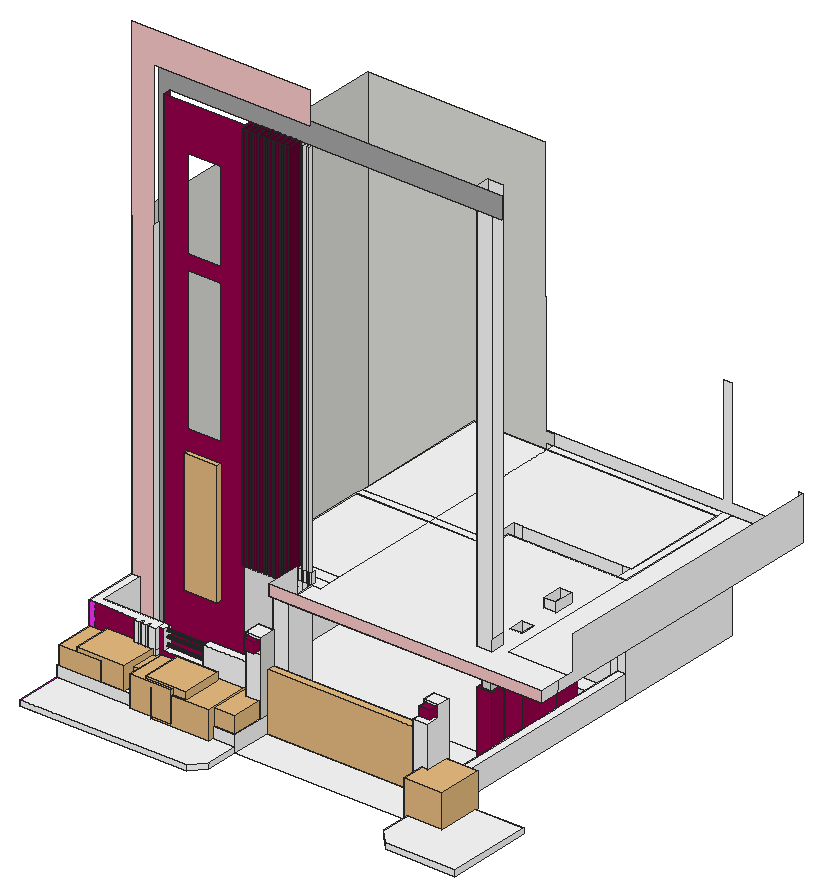
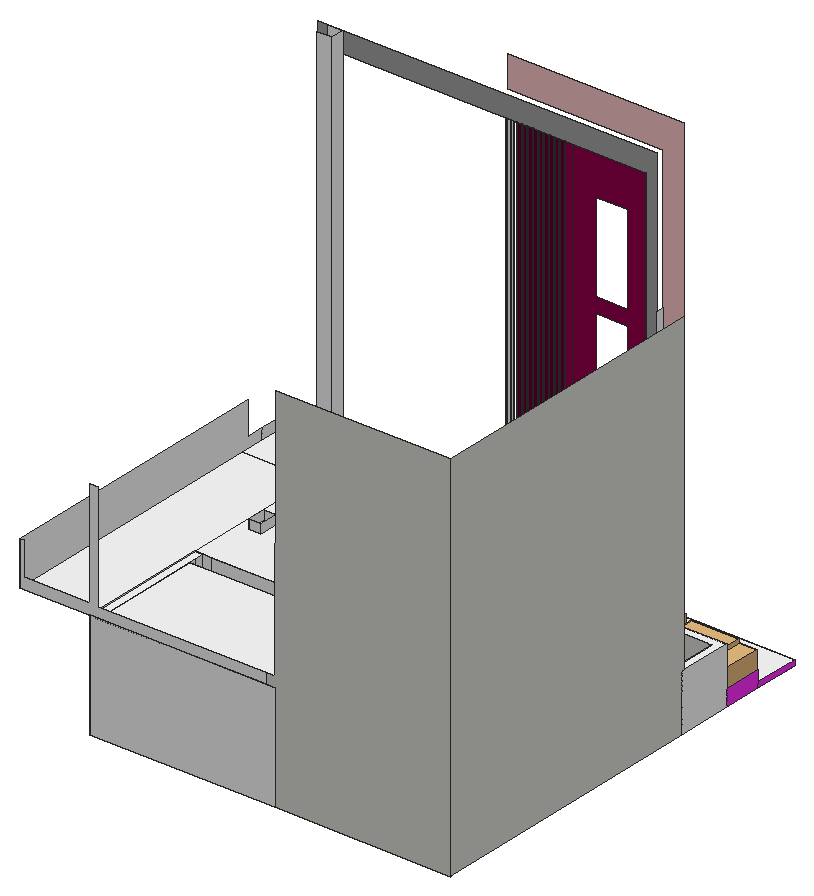
# SketchUp Ruby script. Lengths in inches.
U = 1.inch
M = Sketchup.active_model
def pt(a) = Geom::Point3d.new(a.map { |v| v * U })
def face(e, loops, mat)
  f = e.add_face(loops[0].map { |a| pt(a) })
  loops[1..].each { |l| e.add_face(l.map { |a| pt(a) }).erase! }
  f.material = f.back_material = mat if mat
  f
end
# faces: each face lists its corners as indices into pts; further lists are holes
def faces(e, pts, list, mat = nil) = list.each { |f| face(e, (f[0].is_a?(Array) ? f : [f]).map { |l| l.map { |i| pts[i] } }, mat) }
# xy, xz, yz: faces in a plane at the given z, y or x. An outline is a flat list of corners, or four numbers for a rectangle; further outlines are holes
def ring(l) = l.size == 4 ? [[l[0], l[1]], [l[2], l[1]], [l[2], l[3]], [l[0], l[3]]] : l.each_slice(2).to_a
def flat(e, list, mat, &to3) = list.each { |f| face(e, (f[0].is_a?(Array) ? f : [f]).map { |l| ring(l).map { |u, v| to3.(u, v) } }, mat) }
def xy(e, z, list, mat = nil) = flat(e, list, mat) { |x, y| [x, y, z] }
def xz(e, y, list, mat = nil) = flat(e, list, mat) { |x, z| [x, y, z] }
def yz(e, x, list, mat = nil) = flat(e, list, mat) { |y, z| [x, y, z] }
def lines(e, pts, list) = list.each { |a, b| e.add_line(pt(pts[a]), pt(pts[b])) }
# prism: a flat outline (further loops are holes) pulled along v
def prism(e, loops, v, mat = nil)
  f = face(e, loops, mat); d = Geom::Vector3d.new(v.map { |x| x * U })
  f.pushpull(f.normal.samedirection?(d) ? d.length : -d.length)
end
def box(e, o, s, mat = nil) = prism(e, [[o, [o[0] + s[0], o[1], o[2]], [o[0] + s[0], o[1] + s[1], o[2]], [o[0], o[1] + s[1], o[2]]]], [0, 0, s[2]], mat)
def at(x, y, z, deg = 0) = Geom::Transformation.translation(pt([x, y, z])) * Geom::Transformation.rotation(ORIGIN, Z_AXIS, deg.degrees)
def axes(o, x, y, z) = Geom::Transformation.new([*x, 0, *y, 0, *z, 0, *pt(o).to_a, 1])
def part(name) = M.definitions.add(name)
# library, detail: a bought-in or finely detailed component or shape, given as its bounding box
def library(name, o, s) = part(name).tap { |d| box(d.entities, o, s) }
def detail(e, o, s) = box(e.add_group.entities, o, s)
def put(e, d, t, mat = nil) = e.add_instance(d, t).tap { |i| i.material = mat if mat }
def group(e, t, mat = nil) = e.add_group.tap { |g| g.transformation = t; g.material = mat if mat }.entities
root = M.entities
M.materials.add("A01_Blush_Petal").color = [255, 204, 204]
M.materials.add("Glass_Basic_01").color = [161, 173, 186]
M.materials["Glass_Basic_01"].alpha = 0.25
M.materials.add("K04_Fuchsia_Dream").color = [255, 49, 255]
M.materials.add("L07_Raspberry_Rush").color = [153, 0, 76]
M.materials.add("L08_Velvet_Rose").color = [102, 0, 51]
M.materials.add("M00_Soft_Cloud").color = [255, 255, 255]
M.materials.add("M03_Pewter_Shine").color = [168, 168, 168]
c1 = library("Muhlenbergia dubia 005",[-26.08,-26.3,-0.58],[52.94,50.81,30.73])
c2 = library("Dalea purpurea 005",[-20.94,-21.11,-0.48],[43.54,46.19,36.21])
c3 = library("Sorghum bicolor 003",[-47.6,-43.14,-0.43],[91.82,88.31,82.26])
c4 = library("Door Unit 600mm 300 029",[-15.84,-6.47,-0.18],[31.69,12.97,85.87])
c5 = library("Gate 243 004",[-115.8,-1.69,0],[231.6,3.38,71.78])
c6 = library("Window 109 024",[-19.35,-1.51,-0.23],[38.7,3.02,80.98])
c7 = library("Scabiosa atropurpurea 007",[-28.01,-27.9375,-1.21],[55.43,54.4,41.93])
c8 = library("Group\#30",[0,0,0],[77.46,3.16,80.98])
c9 = library("Window 109 023",[-16.24,-1.39,-0.03],[32.48,2.78,89.27])
xy(root,0,[[199,95.57,377.49,104.57]])
xy(root,0,[[1,0,1,51.18,199,51.18,199,14.31,186.11,0],[1,51.18,199,51.18,199,95.57,193,95.57,193,57.18,7,57.18,7,95.57,1,95.57],[199,51.18,391.74,51.18,391.74,75.08,377.49,75.08,377.49,95.57,199,95.57],[7,57.18,193,57.18,193,86.8,182.05,86.8,182.05,95.57,78.09,95.57,78.09,91.57,69.69,91.57,69.69,95.57,67.875,95.57,67.875,91.57,61.72,91.57,61.72,95.57,59.82,95.57,59.82,91.57,53.61,91.57,53.61,95.57,7,95.57],[397.74,57.18,423.32,89.57],
  [394.03,95.57,405.98,104.57],[10,104.57,396.98,104.57,396.98,153.91,199,153.91,199,125.3,182.05,125.3,182.05,153.91,136,153.91,136,145.91,127,145.91,127,154.91,37,154.91,37,145.91,28,145.91,28,162.91,25,162.91,25,155.3,10,155.3],[182.05,125.3,199,153.91],[28,145.91,37,162.91],[[127,145.91,136,145.91,136,153.91,182.05,153.91,182.05,158.3,199,158.3,199,153.91,396.98,153.91,396.98,184.56,127,184.56],[377.49,163.42,394.03,178.61]],
  [182.05,153.91,199,158.3],[127,184.56,396.98,184.56,396.98,202.8,377.49,202.8,377.49,225.36,396.98,225.36,396.98,250.62,377.49,250.62,377.49,277.78,396.98,277.78,396.98,309.21,127,309.21],[275.24,309.21,396.98,318.21],[127,318.21,136,318.21,136,464.39,257.24,464.39,257.24,318.21,266.24,318.21,266.24,473.39,127,473.39],[136,318.21,257.24,464.39],
  [266.24,354.24,275.24,354.24,275.24,464.39,387.98,464.39,387.98,354.24,396.98,354.24,396.98,473.39,266.24,473.39],[275.24,354.24,387.98,464.39]],"M00_Soft_Cloud")
xy(root,5.18,[[22.22,93.47,50.11,95.57]],"M00_Soft_Cloud")
xy(root,5.26,[[134.27,91.57,178.26,95.57]],"L07_Raspberry_Rush")
xy(root,6,[[1,0,186.11,0,199,14.31,199,51.18,1,51.18],[407.54,0,484.64,0,484.64,95.57,429.32,95.57,429.32,51.18,391.74,51.18,391.74,17.29]],"M00_Soft_Cloud")
xy(root,6.4375,[[275.24,318.21,396.98,335.38]],"M00_Soft_Cloud")
xy(root,9.9,[[134.27,91.57,178.26,95.57]],"L07_Raspberry_Rush")
xy(root,10.95,[[22.22,93.47,50.11,95.57]],"M00_Soft_Cloud")
xy(root,18,[[1,51.18,199,51.18,199,86.8,193,86.8,193,57.18,7,57.18,7,95.57,1,95.57],[[391.74,51.18,429.32,51.18,429.32,95.57,394.03,95.57,394.03,75.08,391.74,75.08],[397.74,57.18,423.32,89.57]],[193,86.8,199,95.57]],"M00_Soft_Cloud")
xy(root,26.96,[[396.98,104.57,405.98,335.38]],"M00_Soft_Cloud")
xy(root,42.23,[[84.75,95.57,128.05,104.57]],"M00_Soft_Cloud")
xy(root,63.54,[[53.61,91.57,59.82,91.57,59.82,95.57,61.72,95.57,61.72,91.57,67.875,91.57,67.875,95.57,69.69,95.57,69.69,91.57,78.09,91.57,78.09,104.57,10,104.57,10,155.3,1,155.3,1,95.57,53.61,95.57],[78.09,95.57,84.75,104.57],[128.05,95.57,182.05,104.57]],"M00_Soft_Cloud")
xy(root,79.13,[[[377.49,163.42,394.03,178.61],[380.49,166.42,391.03,175.61]],[[377.49,202.8,396.98,225.36],[380.49,205.8,393.98,222.36]],[[377.49,250.62,396.98,277.78],[380.49,253.62,393.98,274.78]]],"L07_Raspberry_Rush")
xy(root,84.98,[[184.73,80.77,196.3125,86.8]],"L07_Raspberry_Rush")
xy(root,86.2,[[377.49,75.08,394.03,89.57]],"M00_Soft_Cloud")
xy(root,88.03,[[380.2,80.3125,392.08,89.57]],"L07_Raspberry_Rush")
xy(root,96.56,[[184.73,80.77,196.3125,86.8]],"L07_Raspberry_Rush")
xy(root,97.59,[[380.2,80.3125,392.08,89.57]],"L07_Raspberry_Rush")
xy(root,99.42,[[182.05,86.8,199,104.57],[377.49,89.57,394.03,104.57]],"M00_Soft_Cloud")
xy(root,120,[[182.05,119.76,208,125.3],[[208,119.76,484.6,119.76,484.6,171.91,405.98,171.91,405.98,335.38,275.24,335.38,275.24,309.21,208,309.21,208,158.3,199,158.3,199,125.3,208,125.3],[377.49,163.42,394.03,178.61],[380.49,205.8,393.98,222.36]],[129,148,133,148,133,162.91,135,162.91,135,148,139,148,139,162.91,141,162.91,141,148,145,148,145,162.91,147,162.91,147,148,151,148,151,162.91,153,162.91,153,148,157,148,157,162.91,159,162.91,159,148,163,148,163,162.91,165,162.91,165,148,169,148,169,162.91,171,162.91,171,148,175,148,175,162.91,177,162.91,177,148,181,148,181,162.91,198,162.91,198,158.3,208,158.3,208,171.91,127,171.91,127,162.91,129,162.91],[183,158.3,187,162.91],[189,158.3,193,162.91],
  [195,158.3,198,162.91],[[377.49,163.42,394.03,178.61],[380.49,166.42,391.03,175.61]],[127,171.91,208,184.56],[405.98,171.91,484.6,482.39],[127,184.56,208,309.21],
  [127,309.21,208,318.21],[208,309.21,266.24,318.21],[127,318.21,208,473.39],[208,318.21,266.24,318.21,266.24,354.24,396.98,354.24,396.98,473.39,208,473.39],[396.98,335.38,405.98,482.39],
  [208,473.39,396.98,482.39]],"M00_Soft_Cloud")
xz(root,0,[[1,0,186.11,6],[407.54,0,484.64,6]],"M00_Soft_Cloud")
xz(root,51.18,[[1,6,199,18],[391.74,6,429.32,18]],"M00_Soft_Cloud")
xz(root,57.18,[[7,0,193,18],[397.74,0,423.32,18]],"M00_Soft_Cloud")
xz(root,75.08,[[377.49,0,391.74,0,391.74,18,394.03,18,394.03,86.2,377.49,86.2]],"M00_Soft_Cloud")
xz(root,80.3125,[[380.2,88.03,392.08,97.59]],"L07_Raspberry_Rush")
xz(root,80.77,[[184.73,84.98,196.3125,96.56]],"L07_Raspberry_Rush")
xz(root,86.8,[[182.05,0,193,0,193,18,199,18,199,82.29,182.05,82.29],[[182.05,82.29,199,99.25],[184.73,84.98,196.3125,96.56]],[182.05,99.25,199,99.42]],"M00_Soft_Cloud")
xz(root,89.57,[[397.74,0,405.98,18],[405.98,0,423.32,18],[377.49,86.2,394.03,86.2,394.03,88.03,380.2,88.03,380.2,97.59,394.03,97.59,394.03,99.42,377.49,99.42],[392.08,88.03,394.03,97.59]],"M00_Soft_Cloud")
xz(root,91.57,[[134.27,5.26,178.26,9.9]],"L07_Raspberry_Rush")
xz(root,91.57,[[53.61,0,59.82,63.54],[61.72,0,67.875,63.54],[69.69,0,78.09,63.54]],"M00_Soft_Cloud")
xz(root,93.47,[[22.22,5.18,50.11,10.95]],"M00_Soft_Cloud")
xz(root,95.57,[[1,0,7,18],[1,18,7,63.54]],"K04_Fuchsia_Dream")
xz(root,95.57,[[[7,0,53.61,63.54],[22.22,5.18,50.11,10.95]],[78.09,0,128.05,42.23],[78.09,42.23,84.75,63.54]],"L07_Raspberry_Rush")
xz(root,95.57,[[59.82,0,61.72,63.54],[67.875,0,69.69,63.54],[[128.05,0,182.05,63.54],[134.27,5.26,178.26,9.9]],[193,0,199,18],[394.03,0,429.32,18],
  [429.32,0,484.64,6]],"M00_Soft_Cloud")
xz(root,104.57,[[10,0,10,63.54,84.75,63.54,84.75,42.23,128.05,42.23,128.05,63.54,182.05,63.54,182.05,99.42,199,99.42,199,0],[377.49,0,394.03,99.42]])
xz(root,104.57,[[394.03,0,396.98,26.96],[396.98,0,405.98,26.96]],"M00_Soft_Cloud")
xz(root,119.76,[[182.05,120,484.6,132]],"A01_Blush_Petal")
xz(root,125.3,[[182.05,0,199,120]],"M00_Soft_Cloud")
xz(root,148,[[129,120,133,554.29],[135,120,139,554.29],[141,120,145,554.29],[147,120,151,554.29],[153,120,157,554.29],
  [159,120,163,554.29],[165,120,169,554.29],[171,120,175,554.29],[177,120,181,554.29]],"L08_Velvet_Rose")
xz(root,154.91,[[[37,0,127,554.29],[63.82,229.87,100.49,387.8125],[63.82,71.93,100.49,208.3],[63.82,404,100.49,504.8]]],"L07_Raspberry_Rush")
xz(root,155.3,[[10,0,25,0,25,578.29,199,578.29,199,614.29,1,614.29,1,63.54,10,63.54]],"A01_Blush_Petal")
xz(root,158.3,[[182.05,0,183,132],[183,0,187,120],[187,0,189,132],[189,0,193,120],[193,0,195,132],
  [195,0,198,120],[198,0,199,120],[183,120,187,132],[189,120,193,132],[195,120,198,132]],"M00_Soft_Cloud")
xz(root,162.91,[[127,120,129,554.29],[133,120,135,554.29],[139,120,141,554.29],[145,120,147,554.29],[151,120,153,554.29],
  [157,120,159,554.29],[163,120,165,554.29],[169,120,171,554.29],[175,120,177,554.29],[181,120,183,554.29],
  [187,120,189,554.29],[193,120,195,554.29]],"M00_Soft_Cloud")
xz(root,162.91,[[25,0,37,0,37,554.29,405.98,554.29,405.98,578.29,25,578.29]],"M03_Pewter_Shine")
xz(root,163.42,[[377.49,0,394.03,79.13]],"L07_Raspberry_Rush")
xz(root,163.42,[[377.49,120,394.03,578.29]],"M00_Soft_Cloud")
xz(root,166.42,[[380.49,79.13,391.03,120]])
xz(root,175.61,[[380.49,79.13,391.03,120]])
xz(root,178.61,[[377.49,0,394.03,79.13]],"L07_Raspberry_Rush")
xz(root,178.61,[[377.49,120,394.03,578.29]],"M00_Soft_Cloud")
xz(root,202.8,[[377.49,0,396.98,79.13]],"L07_Raspberry_Rush")
xz(root,205.8,[[380.49,79.13,393.98,120]],"M00_Soft_Cloud")
xz(root,222.36,[[380.49,79.13,393.98,120]],"M00_Soft_Cloud")
xz(root,225.36,[[377.49,0,396.98,79.13]],"L07_Raspberry_Rush")
xz(root,250.62,[[377.49,0,396.98,79.13]],"L07_Raspberry_Rush")
xz(root,253.62,[[380.49,79.13,393.98,129.83]],"M00_Soft_Cloud")
xz(root,274.78,[[380.49,79.13,393.98,129.83]],"M00_Soft_Cloud")
xz(root,277.78,[[377.49,0,396.98,79.13]],"L07_Raspberry_Rush")
xz(root,309.21,[[[127,0,199.33,0,199.33,84,259.24,84,259.24,0,266.24,0,266.24,120,127,120],[139.29,28.04,184.5,84]],[266.24,0,275.24,120]],"M00_Soft_Cloud")
xz(root,318.21,[[127,0,136,120],[257.24,0,266.24,120],[275.24,0,396.98,6.4375]],"M00_Soft_Cloud")
xz(root,335.38,[[275.24,6.4375,328.7,6.4375,328.7,84,357.46,84,357.46,6.4375,387.98,6.4375,387.98,120,275.24,120],[387.98,6.4375,396.98,120],[396.98,26.96,405.98,120]],"M00_Soft_Cloud")
xz(root,354.24,[[266.24,0,275.24,120],[387.98,0,396.98,120]],"M00_Soft_Cloud")
xz(root,473.39,[[127,0,396.98,120]],"M00_Soft_Cloud")
xz(root,482.39,[[1,-0.48,1,419.15,198,419.15,198,264.48,199,264.48,199,131.52,208,131.52,208,120,199,120,199,-0.48]])
xz(root,482.39,[[199,0,405.98,120],[208,120,208,131.52,199,131.52,199,132,396.98,132,396.98,252,405.98,252,405.98,132,480.39,132,480.39,169.29,484.6,169.29,484.6,120]],"M00_Soft_Cloud")
yz(root,1,[[158.3,0,158.3,63.54,155.3,63.54,155.3,419.15,482.39,419.15,482.39,0]])
yz(root,1,[[0,0,51.18,6],[51.18,0,95.57,18]],"K04_Fuchsia_Dream")
yz(root,1,[[95.57,0,158.3,63.54]],"M00_Soft_Cloud")
yz(root,7,[[57.18,0,95.57,18]],"K04_Fuchsia_Dream")
yz(root,10,[[104.57,0,155.3,63.54]],"M00_Soft_Cloud")
yz(root,22.22,[[93.47,5.18,95.57,10.95]],"M00_Soft_Cloud")
yz(root,25,[[155.3,0,162.91,419.15]],"M00_Soft_Cloud")
yz(root,37,[[154.91,0,162.91,554.29]],"L07_Raspberry_Rush")
yz(root,50.11,[[93.47,5.18,95.57,10.95]],"M00_Soft_Cloud")
yz(root,53.61,[[91.57,0,95.57,63.54]],"M00_Soft_Cloud")
yz(root,59.82,[[91.57,0,95.57,63.54]],"M00_Soft_Cloud")
yz(root,61.72,[[91.57,0,95.57,63.54]],"M00_Soft_Cloud")
yz(root,67.875,[[91.57,0,95.57,63.54]],"M00_Soft_Cloud")
yz(root,69.69,[[91.57,0,95.57,63.54]],"M00_Soft_Cloud")
yz(root,78.09,[[91.57,0,95.57,42.23],[91.57,42.23,95.57,63.54]],"M00_Soft_Cloud")
yz(root,84.75,[[[95.57,42.23,104.57,63.54],[100,44.87,99.64,44.93,99.3,45.09,99.02,45.33,98.81,45.63,98.68,45.98,98.65,46.35,98.72,46.71,98.88,47.05,99.12,47.33,99.42,47.54,99.77,47.67,100.14,47.7,100.5,47.63,100.84,47.47,101.12,47.24,101.33,46.93,101.45,46.58,101.49,46.22,101.42,45.85,101.26,45.52,101.02,45.23,100.72,45.02,100.37,44.9],[100,59.74,99.64,59.81,99.3,59.96,99.02,60.2,98.81,60.51,98.68,60.86,98.65,61.22,98.72,61.59,98.88,61.92,99.12,62.21,99.42,62.42,99.77,62.54,100.14,62.57,100.5,62.51,100.84,62.35,101.12,62.11,101.33,61.81,101.45,61.46,101.49,61.09,101.42,60.73,101.26,60.39,101.02,60.11,100.72,59.9,100.37,59.77],[100,53.51,99.64,53.57,99.3,53.73,99.02,53.97,98.81,54.27,98.68,54.62,98.65,54.99,98.72,55.35,98.88,55.6875,99.12,55.97,99.42,56.18,99.77,56.31,100.14,56.34,100.5,56.27,100.84,56.11,101.12,55.875,101.33,55.57,101.45,55.22,101.49,54.85,101.42,54.49,101.26,54.16,101.02,53.875,100.72,53.66,100.37,53.54]]],"M00_Soft_Cloud")
yz(root,127,[[154.91,120,162.91,554.29]],"L07_Raspberry_Rush")
yz(root,127,[[154.91,0,309.21,120],[318.21,0,473.39,120]],"M00_Soft_Cloud")
yz(root,128.05,[[[95.57,42.23,104.57,63.54],[100,44.87,100.37,44.9,100.72,45.02,101.02,45.23,101.26,45.52,101.42,45.85,101.49,46.22,101.45,46.58,101.33,46.93,101.12,47.24,100.84,47.47,100.5,47.63,100.14,47.7,99.77,47.67,99.42,47.54,99.12,47.33,98.88,47.05,98.72,46.71,98.65,46.35,98.68,45.98,98.81,45.63,99.02,45.33,99.3,45.09,99.64,44.93],[100,59.74,100.37,59.77,100.72,59.9,101.02,60.11,101.26,60.39,101.42,60.73,101.49,61.09,101.45,61.46,101.33,61.81,101.12,62.11,100.84,62.35,100.5,62.51,100.14,62.57,99.77,62.54,99.42,62.42,99.12,62.21,98.88,61.92,98.72,61.59,98.65,61.22,98.68,60.86,98.81,60.51,99.02,60.2,99.3,59.96,99.64,59.81],[100,53.51,100.37,53.54,100.72,53.66,101.02,53.875,101.26,54.16,101.42,54.49,101.49,54.85,101.45,55.22,101.33,55.57,101.12,55.875,100.84,56.11,100.5,56.27,100.14,56.34,99.77,56.31,99.42,56.18,99.12,55.97,98.88,55.6875,98.72,55.35,98.65,54.99,98.68,54.62,98.81,54.27,99.02,53.97,99.3,53.73,99.64,53.57]]],"M00_Soft_Cloud")
yz(root,129,[[148,120,162.91,554.29]],"L08_Velvet_Rose")
yz(root,133,[[148,120,162.91,554.29]],"L08_Velvet_Rose")
yz(root,134.27,[[91.57,5.26,95.57,9.9]],"L07_Raspberry_Rush")
yz(root,135,[[148,120,162.91,554.29]],"L08_Velvet_Rose")
yz(root,139,[[148,120,162.91,554.29]],"L08_Velvet_Rose")
yz(root,141,[[148,120,162.91,554.29]],"L08_Velvet_Rose")
yz(root,145,[[148,120,162.91,554.29]],"L08_Velvet_Rose")
yz(root,147,[[148,120,162.91,554.29]],"L08_Velvet_Rose")
yz(root,151,[[148,120,162.91,554.29]],"L08_Velvet_Rose")
yz(root,153,[[148,120,162.91,554.29]],"L08_Velvet_Rose")
yz(root,157,[[148,120,162.91,554.29]],"L08_Velvet_Rose")
yz(root,159,[[148,120,162.91,554.29]],"L08_Velvet_Rose")
yz(root,163,[[148,120,162.91,554.29]],"L08_Velvet_Rose")
yz(root,165,[[148,120,162.91,554.29]],"L08_Velvet_Rose")
yz(root,169,[[148,120,162.91,554.29]],"L08_Velvet_Rose")
yz(root,171,[[148,120,162.91,554.29]],"L08_Velvet_Rose")
yz(root,175,[[148,120,162.91,554.29]],"L08_Velvet_Rose")
yz(root,177,[[148,120,162.91,554.29]],"L08_Velvet_Rose")
yz(root,178.26,[[91.57,5.26,95.57,9.9]],"L07_Raspberry_Rush")
yz(root,181,[[148,120,162.91,554.29]],"L08_Velvet_Rose")
yz(root,182.05,[[86.8,0,95.57,62.66],[125.3,0,125.3,120,119.76,120,119.76,132,158.3,132,158.3,0],[86.8,62.66,95.57,99.42],[95.57,63.54,104.57,99.42]],"M00_Soft_Cloud")
yz(root,183,[[158.3,120,162.91,132]],"M00_Soft_Cloud")
yz(root,184.73,[[80.77,84.98,86.8,96.56]],"L07_Raspberry_Rush")
yz(root,187,[[158.3,120,162.91,132]],"M00_Soft_Cloud")
yz(root,189,[[158.3,120,162.91,554.29]],"M00_Soft_Cloud")
yz(root,193,[[57.18,0,86.8,18],[86.8,0,95.57,18],[158.3,120,162.91,554.29]],"M00_Soft_Cloud")
yz(root,195,[[158.3,120,162.91,554.29]],"M00_Soft_Cloud")
yz(root,196.3125,[[80.77,84.98,86.8,96.56]],"L07_Raspberry_Rush")
yz(root,198,[[158.3,120,162.91,132]],"M00_Soft_Cloud")
yz(root,199,[[95.57,0,104.57,0,104.57,99.42,86.8,99.42,86.8,18,95.57,18]])
yz(root,199,[[14.31,0,51.18,6],[51.18,0,95.57,18],[125.3,0,158.3,120]],"M00_Soft_Cloud")
yz(root,266.24,[[309.21,0,318.21,120],[318.21,0,354.24,120]],"M00_Soft_Cloud")
yz(root,275.24,[[309.21,0,318.21,0,318.21,6.4375,335.38,6.4375,335.38,120,309.21,120]],"M00_Soft_Cloud")
yz(root,377.49,[[75.08,0,75.08,86.2,89.57,86.2,89.57,99.42,104.57,99.42,104.57,0]])
yz(root,377.49,[[163.42,0,178.61,79.13],[202.8,0,225.36,79.13],[250.62,0,277.78,79.13]],"L07_Raspberry_Rush")
yz(root,377.49,[[163.42,120,178.61,578.29]],"M00_Soft_Cloud")
yz(root,380.2,[[80.3125,88.03,89.57,97.59]],"L07_Raspberry_Rush")
yz(root,380.49,[[166.42,79.13,175.61,120]])
yz(root,380.49,[[205.8,79.13,222.36,120],[253.62,79.13,274.78,129.83]],"M00_Soft_Cloud")
yz(root,391.03,[[166.42,79.13,175.61,120]])
yz(root,391.74,[[17.29,0,51.18,6],[51.18,0,75.08,18]],"M00_Soft_Cloud")
yz(root,392.08,[[80.3125,88.03,89.57,97.59]],"L07_Raspberry_Rush")
yz(root,393.98,[[205.8,79.13,222.36,120],[253.62,79.13,274.78,129.83]],"M00_Soft_Cloud")
yz(root,394.03,[[163.42,0,178.61,79.13]],"L07_Raspberry_Rush")
yz(root,394.03,[[95.57,0,104.57,0,104.57,99.42,89.57,99.42,89.57,86.2,75.08,86.2,75.08,18,95.57,18],[163.42,120,178.61,132]],"M00_Soft_Cloud")
yz(root,396.98,[[202.8,26.96,225.36,79.13],[250.62,26.96,277.78,79.13]],"L07_Raspberry_Rush")
yz(root,396.98,[[104.57,0,153.91,26.96],[153.91,0,184.56,26.96],[184.56,0,202.8,26.96],[225.36,0,250.62,26.96],[277.78,0,309.21,26.96],
  [309.21,0,318.21,26.96],[354.24,0,473.39,120],[318.21,6.4375,335.38,26.96]],"M00_Soft_Cloud")
yz(root,397.74,[[57.18,0,89.57,18]],"M00_Soft_Cloud")
yz(root,405.98,[[104.57,0,335.38,26.96],[335.38,0,482.39,120]],"M00_Soft_Cloud")
yz(root,423.32,[[57.18,0,89.57,18]],"M00_Soft_Cloud")
yz(root,429.32,[[51.18,6,95.57,18]],"M00_Soft_Cloud")
yz(root,484.6,[[119.76,120,142.83,132],[142.83,120,482.39,120,482.39,169.29,163.42,169.29,163.42,132,142.83,132]],"M00_Soft_Cloud")
yz(root,484.64,[[0,0,95.57,6]],"M00_Soft_Cloud")
p = [[199,14.31,6],[186.11,0,6],[186.11,0,0],[199,14.31,0],[391.74,17.29,0],[407.54,0,0],
  [407.54,0,6],[391.74,17.29,6],[84.75,99.3,45.09],[84.75,99.64,44.93],[128.05,99.64,44.93],[128.05,99.3,45.09],
  [84.75,100,44.87],[128.05,100,44.87],[84.75,100.37,44.9],[128.05,100.37,44.9],[84.75,100.72,45.02],[128.05,100.72,45.02],
  [84.75,101.02,45.23],[128.05,101.02,45.23],[84.75,99.02,45.33],[128.05,99.02,45.33],[84.75,101.26,45.52],[128.05,101.26,45.52],
  [84.75,98.81,45.63],[128.05,98.81,45.63],[84.75,101.42,45.85],[128.05,101.42,45.85],[84.75,98.68,45.98],[128.05,98.68,45.98],
  [84.75,101.49,46.22],[128.05,101.49,46.22],[84.75,98.65,46.35],[128.05,98.65,46.35],[84.75,101.45,46.58],[128.05,101.45,46.58],
  [84.75,98.72,46.71],[128.05,98.72,46.71],[84.75,101.33,46.93],[128.05,101.33,46.93],[84.75,98.88,47.05],[128.05,98.88,47.05],
  [84.75,101.12,47.24],[128.05,101.12,47.24],[84.75,99.12,47.33],[128.05,99.12,47.33],[84.75,100.84,47.47],[128.05,100.84,47.47],
  [84.75,99.42,47.54],[128.05,99.42,47.54],[84.75,99.77,47.67],[128.05,99.77,47.67],[84.75,100.5,47.63],[128.05,100.5,47.63],
  [84.75,100.14,47.7],[128.05,100.14,47.7],[84.75,99.64,53.57],[84.75,100,53.51],[128.05,100,53.51],[128.05,99.64,53.57],
  [84.75,100.37,53.54],[128.05,100.37,53.54],[84.75,100.72,53.66],[128.05,100.72,53.66],[84.75,99.3,53.73],[128.05,99.3,53.73],
  [84.75,99.02,53.97],[128.05,99.02,53.97],[84.75,101.02,53.875],[128.05,101.02,53.875],[84.75,101.26,54.16],[128.05,101.26,54.16],
  [84.75,98.81,54.27],[128.05,98.81,54.27],[84.75,101.42,54.49],[128.05,101.42,54.49],[84.75,98.68,54.62],[128.05,98.68,54.62],
  [84.75,101.49,54.85],[128.05,101.49,54.85],[84.75,98.65,54.99],[128.05,98.65,54.99],[84.75,101.45,55.22],[128.05,101.45,55.22],
  [84.75,98.72,55.35],[128.05,98.72,55.35],[84.75,101.33,55.57],[128.05,101.33,55.57],[84.75,98.88,55.6875],[128.05,98.88,55.6875],
  [84.75,101.12,55.875],[128.05,101.12,55.875],[84.75,99.12,55.97],[128.05,99.12,55.97],[84.75,100.84,56.11],[128.05,100.84,56.11],
  [84.75,99.42,56.18],[128.05,99.42,56.18],[84.75,100.5,56.27],[128.05,100.5,56.27],[84.75,99.77,56.31],[128.05,99.77,56.31],
  [84.75,100.14,56.34],[128.05,100.14,56.34],[84.75,99.64,59.81],[84.75,100,59.74],[128.05,100,59.74],[128.05,99.64,59.81],
  [84.75,100.37,59.77],[128.05,100.37,59.77],[84.75,99.3,59.96],[128.05,99.3,59.96],[84.75,100.72,59.9],[128.05,100.72,59.9],
  [84.75,101.02,60.11],[128.05,101.02,60.11],[84.75,99.02,60.2],[128.05,99.02,60.2],[84.75,101.26,60.39],[128.05,101.26,60.39],
  [84.75,98.81,60.51],[128.05,98.81,60.51],[84.75,101.42,60.73],[128.05,101.42,60.73],[84.75,98.68,60.86],[128.05,98.68,60.86],
  [84.75,101.49,61.09],[128.05,101.49,61.09],[84.75,98.65,61.22],[128.05,98.65,61.22],[84.75,101.45,61.46],[128.05,101.45,61.46],
  [84.75,98.72,61.59],[128.05,98.72,61.59],[84.75,101.33,61.81],[128.05,101.33,61.81],[84.75,98.88,61.92],[128.05,98.88,61.92],
  [84.75,101.12,62.11],[128.05,101.12,62.11],[84.75,99.12,62.21],[128.05,99.12,62.21],[84.75,100.84,62.35],[128.05,100.84,62.35],
  [84.75,99.42,62.42],[128.05,99.42,62.42],[84.75,100.5,62.51],[128.05,100.5,62.51],[84.75,99.77,62.54],[128.05,99.77,62.54],
  [84.75,100.14,62.57],[128.05,100.14,62.57],[448.07,795.54,0],[448.07,795.54,-0.48],[448.07,1115.02,0],[448.07,1115.02,-0.48],
  [559.5,592.5,0],[559.5,592.5,-0.48],[397.74,89.57,18],[396.98,89.57,18]]
faces(root,p,[[0,1,2,3],[4,5,6,7],[8,9,10,11],[9,12,13,10],[12,14,15,13],[14,16,17,15],[16,18,19,17],[20,8,11,21],
  [18,22,23,19],[24,20,21,25],[22,26,27,23],[28,24,25,29],[26,30,31,27],[32,28,29,33],[30,34,35,31],[36,32,33,37],
  [34,38,39,35],[40,36,37,41],[38,42,43,39],[44,40,41,45],[42,46,47,43],[48,44,45,49],[50,48,49,51],[46,52,53,47],
  [52,54,55,53],[54,50,51,55],[56,57,58,59],[57,60,61,58],[60,62,63,61],[64,56,59,65],[66,64,65,67],[62,68,69,63],
  [68,70,71,69],[72,66,67,73],[70,74,75,71],[76,72,73,77],[74,78,79,75],[80,76,77,81],[78,82,83,79],[84,80,81,85],
  [82,86,87,83],[88,84,85,89],[86,90,91,87],[92,88,89,93],[90,94,95,91],[96,92,93,97],[94,98,99,95],[100,96,97,101],
  [102,100,101,103],[98,102,103,99],[104,105,106,107],[105,108,109,106],[110,104,107,111],[108,112,113,109],[112,114,115,113],[116,110,111,117],
  [114,118,119,115],[120,116,117,121],[118,122,123,119],[124,120,121,125],[122,126,127,123],[128,124,125,129],[126,130,131,127],[132,128,129,133],
  [130,134,135,131],[136,132,133,137],[134,138,139,135],[140,136,137,141],[138,142,143,139],[144,140,141,145],[142,146,147,143],[148,144,145,149],
  [150,148,149,151],[146,150,151,147]],"M00_Soft_Cloud")
lines(root,p,[[152,153],[154,155],[156,157],[158,159]])
put(root,c1,axes([141.51,77.11,0.12],[1.2,0,0],[0,1.2,0],[0,0,1.2]))
put(root,c2,axes([24.52,74.39,0.03],[1.07,0,0],[0,1.07,0],[0,0,1.07]))
put(root,c3,axes([75.08,84.2,-0.23],[0.45201,0,0],[0,0.45201,0],[0,0,0.45201]))
put(root,c4,axes([227.99,310.02,0.02],[1.8094,0,0],[0,0.17072,0],[0,0,0.983]))
put(root,c5,axes([290.19,99.95,-0.02],[0.78771,0,0],[0,2.59374,0],[0,0,0.89]),"Glass_Basic_01")
put(root,c1,axes([165.84,83.13,1.01],[1.15,0,0],[0,1.15,0],[0,0,1.15]))
put(root,c1,axes([405.98,84.0625,4],[0.481,0,0],[0,0.65,0],[0,0,0.455]))
put(root,c3,axes([409.55,74.5,4.17],[0.46248,0,0],[0,0.56885,0],[0,0,0.46248]))
put(root,c6,axes([343.08,335.6,6.66],[0.74297,0,0],[0,1.1792,0],[0,0,0.95784]))
put(root,c7,axes([109.5,67.94,9.09],[0.81,0,0],[0,0.81,0],[0,0,0.81]))
put(root,c7,axes([124.5,70.95,11.11],[0.81,0,0],[0,0.81,0],[0,0,0.81]))
put(root,c1,at(47.8,78.8,12.45))
put(root,c8,axes([139.29,318.5,27.48],[0.58951,0,0],[0,-2.96621,0],[0,0,0.69799]))
put(root,c9,axes([82.17,152.22,71.98],[1.12885,0,0],[0,2.41551,0],[0,0,1.5276]))
